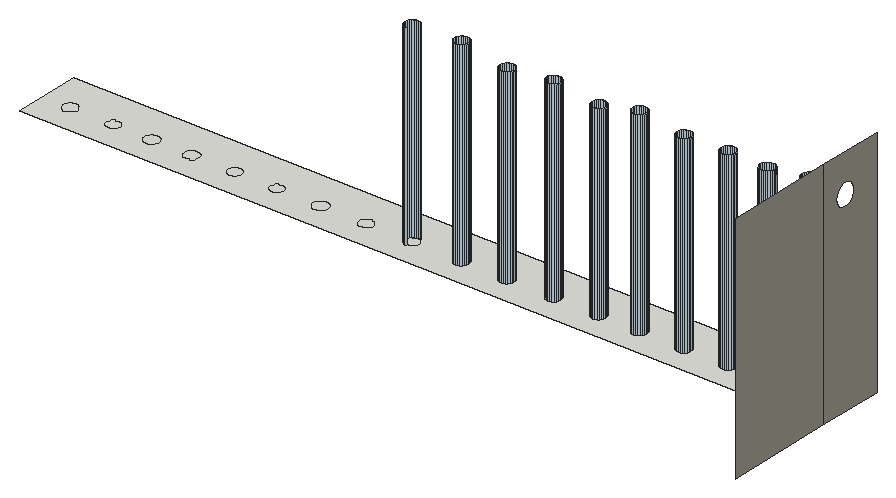
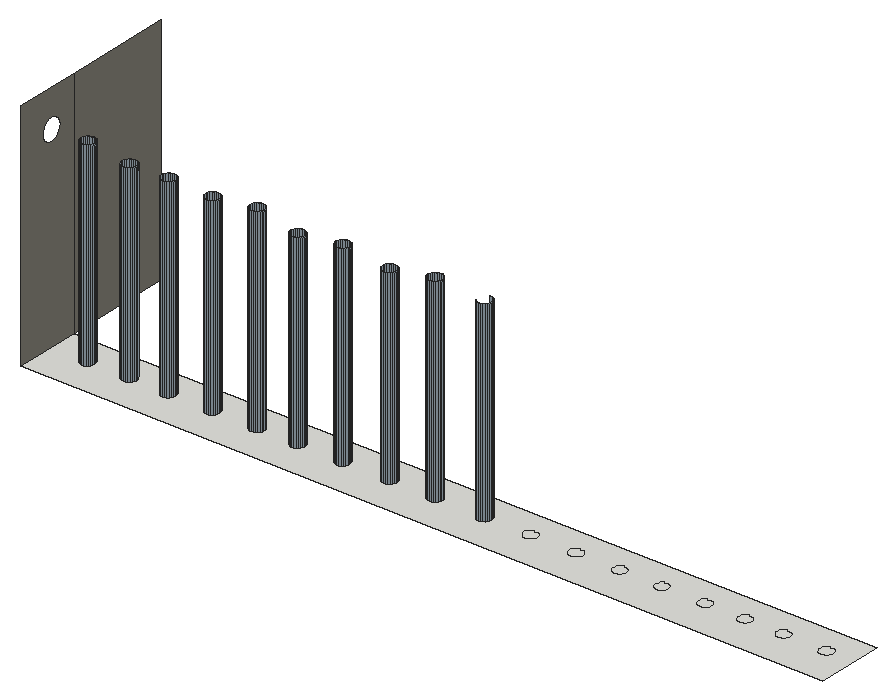
# SketchUp Ruby script. Lengths in inches.
U = 1.inch
M = Sketchup.active_model
def pt(a) = Geom::Point3d.new(a.map { |v| v * U })
def face(e, loops, mat)
  f = e.add_face(loops[0].map { |a| pt(a) })
  loops[1..].each { |l| e.add_face(l.map { |a| pt(a) }).erase! }
  f.material = f.back_material = mat if mat
  f
end
# faces: each face lists its corners as indices into pts; further lists are holes
def faces(e, pts, list, mat = nil) = list.each { |f| face(e, (f[0].is_a?(Array) ? f : [f]).map { |l| l.map { |i| pts[i] } }, mat) }
# xy, xz, yz: faces in a plane at the given z, y or x. An outline is a flat list of corners, or four numbers for a rectangle; further outlines are holes
def ring(l) = l.size == 4 ? [[l[0], l[1]], [l[2], l[1]], [l[2], l[3]], [l[0], l[3]]] : l.each_slice(2).to_a
def flat(e, list, mat, &to3) = list.each { |f| face(e, (f[0].is_a?(Array) ? f : [f]).map { |l| ring(l).map { |u, v| to3.(u, v) } }, mat) }
def xy(e, z, list, mat = nil) = flat(e, list, mat) { |x, y| [x, y, z] }
def xz(e, y, list, mat = nil) = flat(e, list, mat) { |x, z| [x, y, z] }
def yz(e, x, list, mat = nil) = flat(e, list, mat) { |y, z| [x, y, z] }
def lines(e, pts, list) = list.each { |a, b| e.add_line(pt(pts[a]), pt(pts[b])) }
# prism: a flat outline (further loops are holes) pulled along v
def prism(e, loops, v, mat = nil)
  f = face(e, loops, mat); d = Geom::Vector3d.new(v.map { |x| x * U })
  f.pushpull(f.normal.samedirection?(d) ? d.length : -d.length)
end
def box(e, o, s, mat = nil) = prism(e, [[o, [o[0] + s[0], o[1], o[2]], [o[0] + s[0], o[1] + s[1], o[2]], [o[0], o[1] + s[1], o[2]]]], [0, 0, s[2]], mat)
def at(x, y, z, deg = 0) = Geom::Transformation.translation(pt([x, y, z])) * Geom::Transformation.rotation(ORIGIN, Z_AXIS, deg.degrees)
def axes(o, x, y, z) = Geom::Transformation.new([*x, 0, *y, 0, *z, 0, *pt(o).to_a, 1])
def part(name) = M.definitions.add(name)
# library, detail: a bought-in or finely detailed component or shape, given as its bounding box
def library(name, o, s) = part(name).tap { |d| box(d.entities, o, s) }
def detail(e, o, s) = box(e.add_group.entities, o, s)
def put(e, d, t, mat = nil) = e.add_instance(d, t).tap { |i| i.material = mat if mat }
def group(e, t, mat = nil) = e.add_group.tap { |g| g.transformation = t; g.material = mat if mat }.entities
root = M.entities
M.materials.add("[Formica Graystone]").color = [149, 146, 135]
M.materials.add("[Terrazzo Light Blue]").color = [196, 214, 227]
xy(root,2196.1875,[[[746.18,769.97,1870.17,862.78],[1760.72,798.92,1758.15,799.26,1755.75,800.25,1753.7,801.83,1752.12,803.89,1751.125,806.29,1750.79,808.86,1751.125,811.43,1752.12,813.83,1753.7,815.89,1755.75,817.46,1758.15,818.46,1760.72,818.8,1763.3,818.46,1765.69,817.46,1767.75,815.89,1769.33,813.83,1770.32,811.43,1770.66,808.86,1770.32,806.29,1769.33,803.89,1767.75,801.83,1765.69,800.25,1763.3,799.26],[1581.79,798.92,1579.21,799.26,1576.82,800.25,1574.76,801.83,1573.18,803.89,1572.1875,806.29,1571.85,808.86,1572.1875,811.43,1573.18,813.83,1574.76,815.89,1576.82,817.46,1579.21,818.46,1581.79,818.8,1584.36,818.46,1586.75,817.46,1588.8125,815.89,1590.39,813.83,1591.39,811.43,1591.72,808.86,1591.39,806.29,1590.39,803.89,1588.8125,801.83,1586.75,800.25,1584.36,799.26],[1524.85,798.92,1522.28,799.26,1519.88,800.25,1517.82,801.83,1516.24,803.89,1515.25,806.29,1514.91,808.86,1515.25,811.43,1516.24,813.83,1517.82,815.89,1519.88,817.46,1522.28,818.46,1524.85,818.8,1527.42,818.46,1529.82,817.46,1531.875,815.89,1533.45,813.83,1534.45,811.43,1534.79,808.86,1534.45,806.29,1533.45,803.89,1531.875,801.83,1529.82,800.25,1527.42,799.26],[1461.66,798.92,1459.09,799.26,1456.69,800.25,1454.63,801.83,1453.06,803.89,1452.0625,806.29,1451.72,808.86,1452.0625,811.43,1453.06,813.83,1454.63,815.89,1456.69,817.46,1459.09,818.46,1461.66,818.8,1464.23,818.46,1466.63,817.46,1468.6875,815.89,1470.27,813.83,1471.26,811.43,1471.6,808.86,1471.26,806.29,1470.27,803.89,1468.6875,801.83,1466.63,800.25,1464.23,799.26],[1199.35,798.92,1196.78,799.26,1194.38,800.25,1192.32,801.83,1190.74,803.89,1189.75,806.29,1189.41,808.86,1189.75,811.43,1190.74,813.83,1192.32,815.89,1194.38,817.46,1196.78,818.46,1199.35,818.8,1201.92,818.46,1204.32,817.46,1206.375,815.89,1207.95,813.83,1208.95,811.43,1209.29,808.86,1208.95,806.29,1207.95,803.89,1206.375,801.83,1204.32,800.25,1201.92,799.26],[1332.66,798.92,1330.09,799.26,1327.69,800.25,1325.63,801.83,1324.06,803.89,1323.0625,806.29,1322.72,808.86,1323.0625,811.43,1324.06,813.83,1325.63,815.89,1327.69,817.46,1330.09,818.46,1332.66,818.8,1335.23,818.46,1337.63,817.46,1339.6875,815.89,1341.27,813.83,1342.26,811.43,1342.6,808.86,1342.26,806.29,1341.27,803.89,1339.6875,801.83,1337.63,800.25,1335.23,799.26],[785.04,798.92,782.46,799.26,780.07,800.25,778.01,801.83,776.43,803.89,775.4375,806.29,775.1,808.86,775.4375,811.43,776.43,813.83,778.01,815.89,780.07,817.46,782.46,818.46,785.04,818.8,787.61,818.46,790,817.46,792.0625,815.89,793.64,813.83,794.64,811.43,794.97,808.86,794.64,806.29,793.64,803.89,792.0625,801.83,790,800.25,787.61,799.26],[845.1,798.92,842.53,799.26,840.13,800.25,838.07,801.83,836.49,803.89,835.5,806.29,835.16,808.86,835.5,811.43,836.49,813.83,838.07,815.89,840.13,817.46,842.53,818.46,845.1,818.8,847.67,818.46,850.07,817.46,852.125,815.89,853.7,813.83,854.7,811.43,855.04,808.86,854.7,806.29,853.7,803.89,852.125,801.83,850.07,800.25,847.67,799.26],[898.66,798.92,896.09,799.26,893.69,800.25,891.63,801.83,890.06,803.89,889.0625,806.29,888.72,808.86,889.0625,811.43,890.06,813.83,891.63,815.89,893.69,817.46,896.09,818.46,898.66,818.8,901.23,818.46,903.63,817.46,905.6875,815.89,907.27,813.83,908.26,811.43,908.6,808.86,908.26,806.29,907.27,803.89,905.6875,801.83,903.63,800.25,901.23,799.26],[954.66,798.92,952.09,799.26,949.69,800.25,947.63,801.83,946.06,803.89,945.0625,806.29,944.72,808.86,945.0625,811.43,946.06,813.83,947.63,815.89,949.69,817.46,952.09,818.46,954.66,818.8,957.23,818.46,959.63,817.46,961.6875,815.89,963.27,813.83,964.26,811.43,964.6,808.86,964.26,806.29,963.27,803.89,961.6875,801.83,959.63,800.25,957.23,799.26],[1644.29,798.92,1641.71,799.26,1639.32,800.25,1637.26,801.83,1635.68,803.89,1634.6875,806.29,1634.35,808.86,1634.6875,811.43,1635.68,813.83,1637.26,815.89,1639.32,817.46,1641.71,818.46,1644.29,818.8,1646.86,818.46,1649.25,817.46,1651.3125,815.89,1652.89,813.83,1653.89,811.43,1654.22,808.86,1653.89,806.29,1652.89,803.89,1651.3125,801.83,1649.25,800.25,1646.86,799.26],[1015.1,798.92,1012.53,799.26,1010.13,800.25,1008.07,801.83,1006.49,803.89,1005.5,806.29,1005.16,808.86,1005.5,811.43,1006.49,813.83,1008.07,815.89,1010.13,817.46,1012.53,818.46,1015.1,818.8,1017.67,818.46,1020.07,817.46,1022.125,815.89,1023.7,813.83,1024.7,811.43,1025.04,808.86,1024.7,806.29,1023.7,803.89,1022.125,801.83,1020.07,800.25,1017.67,799.26],[1074.1,798.92,1071.53,799.26,1069.13,800.25,1067.07,801.83,1065.49,803.89,1064.5,806.29,1064.16,808.86,1064.5,811.43,1065.49,813.83,1067.07,815.89,1069.13,817.46,1071.53,818.46,1074.1,818.8,1076.67,818.46,1079.07,817.46,1081.125,815.89,1082.7,813.83,1083.7,811.43,1084.04,808.86,1083.7,806.29,1082.7,803.89,1081.125,801.83,1079.07,800.25,1076.67,799.26],[1135.1,798.92,1132.53,799.26,1130.13,800.25,1128.07,801.83,1126.49,803.89,1125.5,806.29,1125.16,808.86,1125.5,811.43,1126.49,813.83,1128.07,815.89,1130.13,817.46,1132.53,818.46,1135.1,818.8,1137.67,818.46,1140.07,817.46,1142.125,815.89,1143.7,813.83,1144.7,811.43,1145.04,808.86,1144.7,806.29,1143.7,803.89,1142.125,801.83,1140.07,800.25,1137.67,799.26],[1818.72,798.92,1816.15,799.26,1813.75,800.25,1811.7,801.83,1810.12,803.89,1809.125,806.29,1808.79,808.86,1809.125,811.43,1810.12,813.83,1811.7,815.89,1813.75,817.46,1816.15,818.46,1818.72,818.8,1821.3,818.46,1823.69,817.46,1825.75,815.89,1827.33,813.83,1828.32,811.43,1828.66,808.86,1828.32,806.29,1827.33,803.89,1825.75,801.83,1823.69,800.25,1821.3,799.26],[1705.97,798.92,1703.4,799.26,1701,800.25,1698.95,801.83,1697.37,803.89,1696.375,806.29,1696.04,808.86,1696.375,811.43,1697.37,813.83,1698.95,815.89,1701,817.46,1703.4,818.46,1705.97,818.8,1708.55,818.46,1710.94,817.46,1713,815.89,1714.58,813.83,1715.57,811.43,1715.91,808.86,1715.57,806.29,1714.58,803.89,1713,801.83,1710.94,800.25,1708.55,799.26],[1396.47,798.92,1393.9,799.26,1391.5,800.25,1389.45,801.83,1387.87,803.89,1386.875,806.29,1386.54,808.86,1386.875,811.43,1387.87,813.83,1389.45,815.89,1391.5,817.46,1393.9,818.46,1396.47,818.8,1399.05,818.46,1401.44,817.46,1403.5,815.89,1405.08,813.83,1406.07,811.43,1406.41,808.86,1406.07,806.29,1405.08,803.89,1403.5,801.83,1401.44,800.25,1399.05,799.26],[1263.54,798.92,1260.96,799.26,1258.57,800.25,1256.51,801.83,1254.93,803.89,1253.9375,806.29,1253.6,808.86,1253.9375,811.43,1254.93,813.83,1256.51,815.89,1258.57,817.46,1260.96,818.46,1263.54,818.8,1266.11,818.46,1268.5,817.46,1270.5625,815.89,1272.14,813.83,1273.14,811.43,1273.47,808.86,1273.14,806.29,1272.14,803.89,1270.5625,801.83,1268.5,800.25,1266.11,799.26]],[785.04,798.92,782.46,799.26,780.07,800.25,778.01,801.83,776.43,803.89,775.4375,806.29,775.1,808.86,775.4375,811.43,776.43,813.83,778.01,815.89,780.07,817.46,782.46,818.46,785.04,818.8,787.61,818.46,790,817.46,792.0625,815.89,793.64,813.83,794.64,811.43,794.97,808.86,794.64,806.29,793.64,803.89,792.0625,801.83,790,800.25,787.61,799.26],[845.1,798.92,842.53,799.26,840.13,800.25,838.07,801.83,836.49,803.89,835.5,806.29,835.16,808.86,835.5,811.43,836.49,813.83,838.07,815.89,840.13,817.46,842.53,818.46,845.1,818.8,847.67,818.46,850.07,817.46,852.125,815.89,853.7,813.83,854.7,811.43,855.04,808.86,854.7,806.29,853.7,803.89,852.125,801.83,850.07,800.25,847.67,799.26],[898.66,798.92,896.09,799.26,893.69,800.25,891.63,801.83,890.06,803.89,889.0625,806.29,888.72,808.86,889.0625,811.43,890.06,813.83,891.63,815.89,893.69,817.46,896.09,818.46,898.66,818.8,901.23,818.46,903.63,817.46,905.6875,815.89,907.27,813.83,908.26,811.43,908.6,808.86,908.26,806.29,907.27,803.89,905.6875,801.83,903.63,800.25,901.23,799.26],[954.66,798.92,952.09,799.26,949.69,800.25,947.63,801.83,946.06,803.89,945.0625,806.29,944.72,808.86,945.0625,811.43,946.06,813.83,947.63,815.89,949.69,817.46,952.09,818.46,954.66,818.8,957.23,818.46,959.63,817.46,961.6875,815.89,963.27,813.83,964.26,811.43,964.6,808.86,964.26,806.29,963.27,803.89,961.6875,801.83,959.63,800.25,957.23,799.26],
  [1015.1,798.92,1012.53,799.26,1010.13,800.25,1008.07,801.83,1006.49,803.89,1005.5,806.29,1005.16,808.86,1005.5,811.43,1006.49,813.83,1008.07,815.89,1010.13,817.46,1012.53,818.46,1015.1,818.8,1017.67,818.46,1020.07,817.46,1022.125,815.89,1023.7,813.83,1024.7,811.43,1025.04,808.86,1024.7,806.29,1023.7,803.89,1022.125,801.83,1020.07,800.25,1017.67,799.26],[1074.1,798.92,1071.53,799.26,1069.13,800.25,1067.07,801.83,1065.49,803.89,1064.5,806.29,1064.16,808.86,1064.5,811.43,1065.49,813.83,1067.07,815.89,1069.13,817.46,1071.53,818.46,1074.1,818.8,1076.67,818.46,1079.07,817.46,1081.125,815.89,1082.7,813.83,1083.7,811.43,1084.04,808.86,1083.7,806.29,1082.7,803.89,1081.125,801.83,1079.07,800.25,1076.67,799.26],[1135.1,798.92,1132.53,799.26,1130.13,800.25,1128.07,801.83,1126.49,803.89,1125.5,806.29,1125.16,808.86,1125.5,811.43,1126.49,813.83,1128.07,815.89,1130.13,817.46,1132.53,818.46,1135.1,818.8,1137.67,818.46,1140.07,817.46,1142.125,815.89,1143.7,813.83,1144.7,811.43,1145.04,808.86,1144.7,806.29,1143.7,803.89,1142.125,801.83,1140.07,800.25,1137.67,799.26],[1199.35,798.92,1196.78,799.26,1194.38,800.25,1192.32,801.83,1190.74,803.89,1189.75,806.29,1189.41,808.86,1189.75,811.43,1190.74,813.83,1192.32,815.89,1194.38,817.46,1196.78,818.46,1199.35,818.8,1201.92,818.46,1204.32,817.46,1206.375,815.89,1207.95,813.83,1208.95,811.43,1209.29,808.86,1208.95,806.29,1207.95,803.89,1206.375,801.83,1204.32,800.25,1201.92,799.26],[1263.54,798.92,1260.96,799.26,1258.57,800.25,1256.51,801.83,1254.93,803.89,1253.9375,806.29,1253.6,808.86,1253.9375,811.43,1254.93,813.83,1256.51,815.89,1258.57,817.46,1260.96,818.46,1263.54,818.8,1266.11,818.46,1268.5,817.46,1270.5625,815.89,1272.14,813.83,1273.14,811.43,1273.47,808.86,1273.14,806.29,1272.14,803.89,1270.5625,801.83,1268.5,800.25,1266.11,799.26],
  [1332.66,798.92,1330.09,799.26,1327.69,800.25,1325.63,801.83,1324.06,803.89,1323.0625,806.29,1322.72,808.86,1323.0625,811.43,1324.06,813.83,1325.63,815.89,1327.69,817.46,1330.09,818.46,1332.66,818.8,1335.23,818.46,1337.63,817.46,1339.6875,815.89,1341.27,813.83,1342.26,811.43,1342.6,808.86,1342.26,806.29,1341.27,803.89,1339.6875,801.83,1337.63,800.25,1335.23,799.26],[1396.47,798.92,1393.9,799.26,1391.5,800.25,1389.45,801.83,1387.87,803.89,1386.875,806.29,1386.54,808.86,1386.875,811.43,1387.87,813.83,1389.45,815.89,1391.5,817.46,1393.9,818.46,1396.47,818.8,1399.05,818.46,1401.44,817.46,1403.5,815.89,1405.08,813.83,1406.07,811.43,1406.41,808.86,1406.07,806.29,1405.08,803.89,1403.5,801.83,1401.44,800.25,1399.05,799.26],[1461.66,798.92,1459.09,799.26,1456.69,800.25,1454.63,801.83,1453.06,803.89,1452.0625,806.29,1451.72,808.86,1452.0625,811.43,1453.06,813.83,1454.63,815.89,1456.69,817.46,1459.09,818.46,1461.66,818.8,1464.23,818.46,1466.63,817.46,1468.6875,815.89,1470.27,813.83,1471.26,811.43,1471.6,808.86,1471.26,806.29,1470.27,803.89,1468.6875,801.83,1466.63,800.25,1464.23,799.26],[1524.85,798.92,1522.28,799.26,1519.88,800.25,1517.82,801.83,1516.24,803.89,1515.25,806.29,1514.91,808.86,1515.25,811.43,1516.24,813.83,1517.82,815.89,1519.88,817.46,1522.28,818.46,1524.85,818.8,1527.42,818.46,1529.82,817.46,1531.875,815.89,1533.45,813.83,1534.45,811.43,1534.79,808.86,1534.45,806.29,1533.45,803.89,1531.875,801.83,1529.82,800.25,1527.42,799.26],[1581.79,798.92,1579.21,799.26,1576.82,800.25,1574.76,801.83,1573.18,803.89,1572.1875,806.29,1571.85,808.86,1572.1875,811.43,1573.18,813.83,1574.76,815.89,1576.82,817.46,1579.21,818.46,1581.79,818.8,1584.36,818.46,1586.75,817.46,1588.8125,815.89,1590.39,813.83,1591.39,811.43,1591.72,808.86,1591.39,806.29,1590.39,803.89,1588.8125,801.83,1586.75,800.25,1584.36,799.26],
  [1644.29,798.92,1641.71,799.26,1639.32,800.25,1637.26,801.83,1635.68,803.89,1634.6875,806.29,1634.35,808.86,1634.6875,811.43,1635.68,813.83,1637.26,815.89,1639.32,817.46,1641.71,818.46,1644.29,818.8,1646.86,818.46,1649.25,817.46,1651.3125,815.89,1652.89,813.83,1653.89,811.43,1654.22,808.86,1653.89,806.29,1652.89,803.89,1651.3125,801.83,1649.25,800.25,1646.86,799.26],[1705.97,798.92,1703.4,799.26,1701,800.25,1698.95,801.83,1697.37,803.89,1696.375,806.29,1696.04,808.86,1696.375,811.43,1697.37,813.83,1698.95,815.89,1701,817.46,1703.4,818.46,1705.97,818.8,1708.55,818.46,1710.94,817.46,1713,815.89,1714.58,813.83,1715.57,811.43,1715.91,808.86,1715.57,806.29,1714.58,803.89,1713,801.83,1710.94,800.25,1708.55,799.26],[1760.72,798.92,1758.15,799.26,1755.75,800.25,1753.7,801.83,1752.12,803.89,1751.125,806.29,1750.79,808.86,1751.125,811.43,1752.12,813.83,1753.7,815.89,1755.75,817.46,1758.15,818.46,1760.72,818.8,1763.3,818.46,1765.69,817.46,1767.75,815.89,1769.33,813.83,1770.32,811.43,1770.66,808.86,1770.32,806.29,1769.33,803.89,1767.75,801.83,1765.69,800.25,1763.3,799.26],[1818.72,798.92,1816.15,799.26,1813.75,800.25,1811.7,801.83,1810.12,803.89,1809.125,806.29,1808.79,808.86,1809.125,811.43,1810.12,813.83,1811.7,815.89,1813.75,817.46,1816.15,818.46,1818.72,818.8,1821.3,818.46,1823.69,817.46,1825.75,815.89,1827.33,813.83,1828.32,811.43,1828.66,808.86,1828.32,806.29,1827.33,803.89,1825.75,801.83,1823.69,800.25,1821.3,799.26]])
yz(root,1870.17,[[617.28,2196.1875,769.97,2522.1875],[[769.97,2196.1875,862.78,2522.1875],[808.34,2453.16,812.38,2453.6875,816.15,2455.25,819.39,2457.73,821.87,2460.97,823.43,2464.74,823.96,2468.78,823.43,2472.82,821.87,2476.59,819.39,2479.83,816.15,2482.3125,812.38,2483.875,808.34,2484.41,804.29,2483.875,800.53,2482.3125,797.29,2479.83,794.81,2476.59,793.25,2472.82,792.71,2468.78,793.25,2464.74,794.81,2460.97,797.29,2457.73,800.53,2455.25,804.29,2453.6875]]],"[Formica Graystone]")
p = [[1260.96,799.26,2196.1875],[1263.54,798.92,2196.1875],[1263.54,798.92,2468.78],[1260.96,799.26,2468.78],[1330.09,799.26,2196.1875],[1332.66,798.92,2196.1875],
  [1332.66,798.92,2472.82],[1330.09,799.26,2472.82],[1335.23,799.26,2196.1875],[1335.23,799.26,2472.82],[1393.9,799.26,2196.1875],[1396.47,798.92,2196.1875],
  [1396.47,798.92,2461.125],[1393.9,799.26,2461.125],[1399.05,799.26,2196.1875],[1399.05,799.26,2461.125],[1459.09,799.26,2196.1875],[1461.66,798.92,2196.1875],
  [1461.66,798.92,2468.78],[1459.09,799.26,2468.78],[1464.23,799.26,2196.1875],[1464.23,799.26,2468.78],[1522.28,799.26,2196.1875],[1524.85,798.92,2196.1875],
  [1524.85,798.92,2460.4375],[1522.28,799.26,2460.4375],[1527.42,799.26,2196.1875],[1527.42,799.26,2460.4375],[1579.21,799.26,2196.1875],[1581.79,798.92,2196.1875],
  [1581.79,798.92,2472.82],[1579.21,799.26,2472.82],[1584.36,799.26,2196.1875],[1584.36,799.26,2472.82],[1641.71,799.26,2196.1875],[1644.29,798.92,2196.1875],
  [1644.29,798.92,2464.4375],[1641.71,799.26,2464.4375],[1646.86,799.26,2196.1875],[1646.86,799.26,2464.4375],[1703.4,799.26,2196.1875],[1705.97,798.92,2196.1875],
  [1705.97,798.92,2466.1875],[1703.4,799.26,2466.1875],[1708.55,799.26,2196.1875],[1708.55,799.26,2466.1875],[1758.15,799.26,2196.1875],[1760.72,798.92,2196.1875],
  [1760.72,798.92,2464.74],[1758.15,799.26,2464.74],[1763.3,799.26,2196.1875],[1763.3,799.26,2464.74],[1816.15,799.26,2196.1875],[1818.72,798.92,2196.1875],
  [1818.72,798.92,2472.9375],[1816.15,799.26,2472.9375],[1821.3,799.26,2196.1875],[1821.3,799.26,2472.9375],[1258.57,800.25,2196.1875],[1258.57,800.25,2468.78],
  [1327.69,800.25,2196.1875],[1327.69,800.25,2472.82],[1337.63,800.25,2196.1875],[1337.63,800.25,2472.82],[1391.5,800.25,2196.1875],[1391.5,800.25,2461.125],
  [1401.44,800.25,2196.1875],[1401.44,800.25,2461.125],[1456.69,800.25,2196.1875],[1456.69,800.25,2468.78],[1466.63,800.25,2196.1875],[1466.63,800.25,2468.78],
  [1519.88,800.25,2196.1875],[1519.88,800.25,2460.4375],[1529.82,800.25,2196.1875],[1529.82,800.25,2460.4375],[1576.82,800.25,2196.1875],[1576.82,800.25,2472.82],
  [1586.75,800.25,2196.1875],[1586.75,800.25,2472.82],[1639.32,800.25,2196.1875],[1639.32,800.25,2464.4375],[1649.25,800.25,2196.1875],[1649.25,800.25,2464.4375],
  [1701,800.25,2196.1875],[1701,800.25,2466.1875],[1710.94,800.25,2196.1875],[1710.94,800.25,2466.1875],[1755.75,800.25,2196.1875],[1755.75,800.25,2464.74],
  [1765.69,800.25,2196.1875],[1765.69,800.25,2464.74],[1813.75,800.25,2196.1875],[1813.75,800.25,2472.9375],[1823.69,800.25,2196.1875],[1823.69,800.25,2472.9375],
  [1256.51,801.83,2196.1875],[1256.51,801.83,2468.78],[1325.63,801.83,2196.1875],[1325.63,801.83,2472.82],[1339.6875,801.83,2196.1875],[1339.6875,801.83,2472.82],
  [1389.45,801.83,2196.1875],[1389.45,801.83,2461.125],[1403.5,801.83,2196.1875],[1403.5,801.83,2461.125],[1454.63,801.83,2196.1875],[1454.63,801.83,2468.78],
  [1468.6875,801.83,2196.1875],[1468.6875,801.83,2468.78],[1517.82,801.83,2196.1875],[1517.82,801.83,2460.4375],[1531.875,801.83,2196.1875],[1531.875,801.83,2460.4375],
  [1574.76,801.83,2196.1875],[1574.76,801.83,2472.82],[1588.8125,801.83,2196.1875],[1588.8125,801.83,2472.82],[1637.26,801.83,2196.1875],[1637.26,801.83,2464.4375],
  [1651.3125,801.83,2196.1875],[1651.3125,801.83,2464.4375],[1698.95,801.83,2196.1875],[1698.95,801.83,2466.1875],[1713,801.83,2196.1875],[1713,801.83,2466.1875],
  [1753.7,801.83,2196.1875],[1753.7,801.83,2464.74],[1767.75,801.83,2196.1875],[1767.75,801.83,2464.74],[1811.7,801.83,2196.1875],[1811.7,801.83,2472.9375],
  [1825.75,801.83,2196.1875],[1825.75,801.83,2472.9375],[1254.93,803.89,2196.1875],[1254.93,803.89,2468.78],[1324.06,803.89,2196.1875],[1324.06,803.89,2472.82],
  [1341.27,803.89,2196.1875],[1341.27,803.89,2472.82],[1387.87,803.89,2196.1875],[1387.87,803.89,2461.125],[1405.08,803.89,2196.1875],[1405.08,803.89,2461.125],
  [1453.06,803.89,2196.1875],[1453.06,803.89,2468.78],[1470.27,803.89,2196.1875],[1470.27,803.89,2468.78],[1516.24,803.89,2196.1875],[1516.24,803.89,2460.4375],
  [1533.45,803.89,2196.1875],[1533.45,803.89,2460.4375],[1573.18,803.89,2196.1875],[1573.18,803.89,2472.82],[1590.39,803.89,2196.1875],[1590.39,803.89,2472.82],
  [1635.68,803.89,2196.1875],[1635.68,803.89,2464.4375],[1652.89,803.89,2196.1875],[1652.89,803.89,2464.4375],[1697.37,803.89,2196.1875],[1697.37,803.89,2466.1875],
  [1714.58,803.89,2196.1875],[1714.58,803.89,2466.1875],[1752.12,803.89,2196.1875],[1752.12,803.89,2464.74],[1769.33,803.89,2196.1875],[1769.33,803.89,2464.74],
  [1810.12,803.89,2196.1875],[1810.12,803.89,2472.9375],[1827.33,803.89,2196.1875],[1827.33,803.89,2472.9375],[1253.9375,806.29,2196.1875],[1253.9375,806.29,2468.78],
  [1323.0625,806.29,2196.1875],[1323.0625,806.29,2472.82],[1342.26,806.29,2196.1875],[1342.26,806.29,2472.82],[1386.875,806.29,2196.1875],[1386.875,806.29,2461.125],
  [1406.07,806.29,2196.1875],[1406.07,806.29,2461.125],[1452.0625,806.29,2196.1875],[1452.0625,806.29,2468.78],[1471.26,806.29,2196.1875],[1471.26,806.29,2468.78],
  [1515.25,806.29,2196.1875],[1515.25,806.29,2460.4375],[1534.45,806.29,2196.1875],[1534.45,806.29,2460.4375],[1572.1875,806.29,2196.1875],[1572.1875,806.29,2472.82],
  [1591.39,806.29,2196.1875],[1591.39,806.29,2472.82],[1634.6875,806.29,2196.1875],[1634.6875,806.29,2464.4375],[1653.89,806.29,2196.1875],[1653.89,806.29,2464.4375],
  [1696.375,806.29,2196.1875],[1696.375,806.29,2466.1875],[1715.57,806.29,2196.1875],[1715.57,806.29,2466.1875],[1751.125,806.29,2196.1875],[1751.125,806.29,2464.74],
  [1770.32,806.29,2196.1875],[1770.32,806.29,2464.74],[1809.125,806.29,2196.1875],[1809.125,806.29,2472.9375],[1828.32,806.29,2196.1875],[1828.32,806.29,2472.9375],
  [1253.6,808.86,2196.1875],[1253.6,808.86,2468.78],[1322.72,808.86,2196.1875],[1322.72,808.86,2472.82],[1342.6,808.86,2196.1875],[1342.6,808.86,2472.82],
  [1386.54,808.86,2196.1875],[1386.54,808.86,2461.125],[1406.41,808.86,2196.1875],[1406.41,808.86,2461.125],[1451.72,808.86,2196.1875],[1451.72,808.86,2468.78],
  [1471.6,808.86,2196.1875],[1471.6,808.86,2468.78],[1514.91,808.86,2196.1875],[1514.91,808.86,2460.4375],[1534.79,808.86,2196.1875],[1534.79,808.86,2460.4375],
  [1571.85,808.86,2196.1875],[1571.85,808.86,2472.82],[1591.72,808.86,2196.1875],[1591.72,808.86,2472.82],[1634.35,808.86,2196.1875],[1634.35,808.86,2464.4375],
  [1654.22,808.86,2196.1875],[1654.22,808.86,2464.4375],[1696.04,808.86,2196.1875],[1696.04,808.86,2466.1875],[1715.91,808.86,2196.1875],[1715.91,808.86,2466.1875],
  [1750.79,808.86,2196.1875],[1750.79,808.86,2464.74],[1770.66,808.86,2196.1875],[1770.66,808.86,2464.74],[1808.79,808.86,2196.1875],[1808.79,808.86,2472.9375],
  [1828.66,808.86,2196.1875],[1828.66,808.86,2472.9375],[1253.9375,811.43,2196.1875],[1253.9375,811.43,2468.78],[1323.0625,811.43,2196.1875],[1323.0625,811.43,2472.82],
  [1342.26,811.43,2196.1875],[1342.26,811.43,2472.82],[1386.875,811.43,2196.1875],[1386.875,811.43,2461.125],[1406.07,811.43,2196.1875],[1406.07,811.43,2461.125],
  [1452.0625,811.43,2196.1875],[1452.0625,811.43,2468.78],[1471.26,811.43,2196.1875],[1471.26,811.43,2468.78],[1515.25,811.43,2196.1875],[1515.25,811.43,2460.4375],
  [1534.45,811.43,2196.1875],[1534.45,811.43,2460.4375],[1572.1875,811.43,2196.1875],[1572.1875,811.43,2472.82],[1591.39,811.43,2196.1875],[1591.39,811.43,2472.82],
  [1634.6875,811.43,2196.1875],[1634.6875,811.43,2464.4375],[1653.89,811.43,2196.1875],[1653.89,811.43,2464.4375],[1696.375,811.43,2196.1875],[1696.375,811.43,2466.1875],
  [1715.57,811.43,2196.1875],[1715.57,811.43,2466.1875],[1751.125,811.43,2196.1875],[1751.125,811.43,2464.74],[1770.32,811.43,2196.1875],[1770.32,811.43,2464.74],
  [1809.125,811.43,2196.1875],[1809.125,811.43,2472.9375],[1828.32,811.43,2196.1875],[1828.32,811.43,2472.9375],[1254.93,813.83,2196.1875],[1254.93,813.83,2468.78],
  [1324.06,813.83,2196.1875],[1324.06,813.83,2472.82],[1341.27,813.83,2196.1875],[1341.27,813.83,2472.82],[1387.87,813.83,2196.1875],[1387.87,813.83,2461.125],
  [1405.08,813.83,2196.1875],[1405.08,813.83,2461.125],[1453.06,813.83,2196.1875],[1453.06,813.83,2468.78],[1470.27,813.83,2196.1875],[1470.27,813.83,2468.78],
  [1516.24,813.83,2196.1875],[1516.24,813.83,2460.4375],[1533.45,813.83,2196.1875],[1533.45,813.83,2460.4375],[1573.18,813.83,2196.1875],[1573.18,813.83,2472.82],
  [1590.39,813.83,2196.1875],[1590.39,813.83,2472.82],[1635.68,813.83,2196.1875],[1635.68,813.83,2464.4375],[1652.89,813.83,2196.1875],[1652.89,813.83,2464.4375],
  [1697.37,813.83,2196.1875],[1697.37,813.83,2466.1875],[1714.58,813.83,2196.1875],[1714.58,813.83,2466.1875],[1752.12,813.83,2196.1875],[1752.12,813.83,2464.74],
  [1769.33,813.83,2196.1875],[1769.33,813.83,2464.74],[1810.12,813.83,2196.1875],[1810.12,813.83,2472.9375],[1827.33,813.83,2196.1875],[1827.33,813.83,2472.9375],
  [1256.51,815.89,2196.1875],[1256.51,815.89,2468.78],[1325.63,815.89,2196.1875],[1325.63,815.89,2472.82],[1339.6875,815.89,2196.1875],[1339.6875,815.89,2472.82],
  [1389.45,815.89,2196.1875],[1389.45,815.89,2461.125],[1403.5,815.89,2196.1875],[1403.5,815.89,2461.125],[1454.63,815.89,2196.1875],[1454.63,815.89,2468.78],
  [1468.6875,815.89,2196.1875],[1468.6875,815.89,2468.78],[1517.82,815.89,2196.1875],[1517.82,815.89,2460.4375],[1531.875,815.89,2196.1875],[1531.875,815.89,2460.4375],
  [1574.76,815.89,2196.1875],[1574.76,815.89,2472.82],[1588.8125,815.89,2196.1875],[1588.8125,815.89,2472.82],[1637.26,815.89,2196.1875],[1637.26,815.89,2464.4375],
  [1651.3125,815.89,2196.1875],[1651.3125,815.89,2464.4375],[1698.95,815.89,2196.1875],[1698.95,815.89,2466.1875],[1713,815.89,2196.1875],[1713,815.89,2466.1875],
  [1753.7,815.89,2196.1875],[1753.7,815.89,2464.74],[1767.75,815.89,2196.1875],[1767.75,815.89,2464.74],[1811.7,815.89,2196.1875],[1811.7,815.89,2472.9375],
  [1825.75,815.89,2196.1875],[1825.75,815.89,2472.9375],[1258.57,817.46,2196.1875],[1258.57,817.46,2468.78],[1270.5625,815.89,2196.1875],[1268.5,817.46,2196.1875],
  [1268.5,817.46,2468.78],[1270.5625,815.89,2468.78],[1327.69,817.46,2196.1875],[1327.69,817.46,2472.82],[1337.63,817.46,2196.1875],[1337.63,817.46,2472.82],
  [1391.5,817.46,2196.1875],[1391.5,817.46,2461.125],[1401.44,817.46,2196.1875],[1401.44,817.46,2461.125],[1456.69,817.46,2196.1875],[1456.69,817.46,2468.78],
  [1466.63,817.46,2196.1875],[1466.63,817.46,2468.78],[1519.88,817.46,2196.1875],[1519.88,817.46,2460.4375],[1529.82,817.46,2196.1875],[1529.82,817.46,2460.4375],
  [1576.82,817.46,2196.1875],[1576.82,817.46,2472.82],[1586.75,817.46,2196.1875],[1586.75,817.46,2472.82],[1639.32,817.46,2196.1875],[1639.32,817.46,2464.4375],
  [1649.25,817.46,2196.1875],[1649.25,817.46,2464.4375],[1701,817.46,2196.1875],[1701,817.46,2466.1875],[1710.94,817.46,2196.1875],[1710.94,817.46,2466.1875],
  [1755.75,817.46,2196.1875],[1755.75,817.46,2464.74],[1765.69,817.46,2196.1875],[1765.69,817.46,2464.74],[1813.75,817.46,2196.1875],[1813.75,817.46,2472.9375],
  [1823.69,817.46,2196.1875],[1823.69,817.46,2472.9375],[1260.96,818.46,2196.1875],[1260.96,818.46,2468.78],[1266.11,818.46,2196.1875],[1266.11,818.46,2468.78],
  [1330.09,818.46,2196.1875],[1330.09,818.46,2472.82],[1335.23,818.46,2196.1875],[1335.23,818.46,2472.82],[1393.9,818.46,2196.1875],[1393.9,818.46,2461.125],
  [1399.05,818.46,2196.1875],[1399.05,818.46,2461.125],[1459.09,818.46,2196.1875],[1459.09,818.46,2468.78],[1464.23,818.46,2196.1875],[1464.23,818.46,2468.78],
  [1522.28,818.46,2196.1875],[1522.28,818.46,2460.4375],[1527.42,818.46,2196.1875],[1527.42,818.46,2460.4375],[1579.21,818.46,2196.1875],[1579.21,818.46,2472.82],
  [1584.36,818.46,2196.1875],[1584.36,818.46,2472.82],[1641.71,818.46,2196.1875],[1641.71,818.46,2464.4375],[1646.86,818.46,2196.1875],[1646.86,818.46,2464.4375],
  [1703.4,818.46,2196.1875],[1703.4,818.46,2466.1875],[1708.55,818.46,2196.1875],[1708.55,818.46,2466.1875],[1758.15,818.46,2196.1875],[1758.15,818.46,2464.74],
  [1763.3,818.46,2196.1875],[1763.3,818.46,2464.74],[1816.15,818.46,2196.1875],[1816.15,818.46,2472.9375],[1821.3,818.46,2196.1875],[1821.3,818.46,2472.9375],
  [1263.54,818.8,2196.1875],[1263.54,818.8,2468.78],[1332.66,818.8,2196.1875],[1332.66,818.8,2472.82],[1396.47,818.8,2196.1875],[1396.47,818.8,2461.125],
  [1461.66,818.8,2196.1875],[1461.66,818.8,2468.78],[1524.85,818.8,2196.1875],[1524.85,818.8,2460.4375],[1581.79,818.8,2196.1875],[1581.79,818.8,2472.82],
  [1644.29,818.8,2196.1875],[1644.29,818.8,2464.4375],[1705.97,818.8,2196.1875],[1705.97,818.8,2466.1875],[1760.72,818.8,2196.1875],[1760.72,818.8,2464.74],
  [1818.72,818.8,2196.1875],[1818.72,818.8,2472.9375]]
faces(root,p,[[0,1,2,3],[4,5,6,7],[5,8,9,6],[10,11,12,13],[11,14,15,12],[16,17,18,19],[17,20,21,18],[22,23,24,25],
  [23,26,27,24],[28,29,30,31],[29,32,33,30],[34,35,36,37],[35,38,39,36],[40,41,42,43],[41,44,45,42],[46,47,48,49],
  [47,50,51,48],[52,53,54,55],[53,56,57,54],[58,0,3,59],[60,4,7,61],[8,62,63,9],[64,10,13,65],[14,66,67,15],
  [68,16,19,69],[20,70,71,21],[72,22,25,73],[26,74,75,27],[76,28,31,77],[32,78,79,33],[80,34,37,81],[38,82,83,39],
  [84,40,43,85],[44,86,87,45],[88,46,49,89],[50,90,91,51],[92,52,55,93],[56,94,95,57],[96,58,59,97],[98,60,61,99],
  [62,100,101,63],[102,64,65,103],[66,104,105,67],[106,68,69,107],[70,108,109,71],[110,72,73,111],[74,112,113,75],[114,76,77,115],
  [78,116,117,79],[118,80,81,119],[82,120,121,83],[122,84,85,123],[86,124,125,87],[126,88,89,127],[90,128,129,91],[130,92,93,131],
  [94,132,133,95],[134,96,97,135],[136,98,99,137],[100,138,139,101],[140,102,103,141],[104,142,143,105],[144,106,107,145],[108,146,147,109],
  [148,110,111,149],[112,150,151,113],[152,114,115,153],[116,154,155,117],[156,118,119,157],[120,158,159,121],[160,122,123,161],[124,162,163,125],
  [164,126,127,165],[128,166,167,129],[168,130,131,169],[132,170,171,133],[172,134,135,173],[174,136,137,175],[138,176,177,139],[178,140,141,179],
  [142,180,181,143],[182,144,145,183],[146,184,185,147],[186,148,149,187],[150,188,189,151],[190,152,153,191],[154,192,193,155],[194,156,157,195],
  [158,196,197,159],[198,160,161,199],[162,200,201,163],[202,164,165,203],[166,204,205,167],[206,168,169,207],[170,208,209,171],[210,172,173,211],
  [212,174,175,213],[176,214,215,177],[216,178,179,217],[180,218,219,181],[220,182,183,221],[184,222,223,185],[224,186,187,225],[188,226,227,189],
  [228,190,191,229],[192,230,231,193],[232,194,195,233],[196,234,235,197],[236,198,199,237],[200,238,239,201],[240,202,203,241],[204,242,243,205],
  [244,206,207,245],[208,246,247,209],[248,210,211,249],[250,212,213,251],[214,252,253,215],[254,216,217,255],[218,256,257,219],[258,220,221,259],
  [222,260,261,223],[262,224,225,263],[226,264,265,227],[266,228,229,267],[230,268,269,231],[270,232,233,271],[234,272,273,235],[274,236,237,275],
  [238,276,277,239],[278,240,241,279],[242,280,281,243],[282,244,245,283],[246,284,285,247],[286,248,249,287],[288,250,251,289],[252,290,291,253],
  [292,254,255,293],[256,294,295,257],[296,258,259,297],[260,298,299,261],[300,262,263,301],[264,302,303,265],[304,266,267,305],[268,306,307,269],
  [308,270,271,309],[272,310,311,273],[312,274,275,313],[276,314,315,277],[316,278,279,317],[280,318,319,281],[320,282,283,321],[284,322,323,285],
  [324,286,287,325],[326,288,289,327],[290,328,329,291],[330,292,293,331],[294,332,333,295],[334,296,297,335],[298,336,337,299],[338,300,301,339],
  [302,340,341,303],[342,304,305,343],[306,344,345,307],[346,308,309,347],[310,348,349,311],[350,312,313,351],[314,352,353,315],[354,316,317,355],
  [318,356,357,319],[358,320,321,359],[322,360,361,323],[362,324,325,363],[364,365,366,367],[368,326,327,369],[328,370,371,329],[372,330,331,373],
  [332,374,375,333],[376,334,335,377],[336,378,379,337],[380,338,339,381],[340,382,383,341],[384,342,343,385],[344,386,387,345],[388,346,347,389],
  [348,390,391,349],[392,350,351,393],[352,394,395,353],[396,354,355,397],[356,398,399,357],[400,358,359,401],[360,402,403,361],[404,362,363,405],
  [365,406,407,366],[408,368,369,409],[370,410,411,371],[412,372,373,413],[374,414,415,375],[416,376,377,417],[378,418,419,379],[420,380,381,421],
  [382,422,423,383],[424,384,385,425],[386,426,427,387],[428,388,389,429],[390,430,431,391],[432,392,393,433],[394,434,435,395],[436,396,397,437],
  [398,438,439,399],[440,400,401,441],[402,442,443,403],[444,404,405,445],[406,444,445,407],[446,408,409,447],[410,446,447,411],[448,412,413,449],
  [414,448,449,415],[450,416,417,451],[418,450,451,419],[452,420,421,453],[422,452,453,423],[454,424,425,455],[426,454,455,427],[456,428,429,457],
  [430,456,457,431],[458,432,433,459],[434,458,459,435],[460,436,437,461],[438,460,461,439],[462,440,441,463],[442,462,463,443]],"[Terrazzo Light Blue]")
